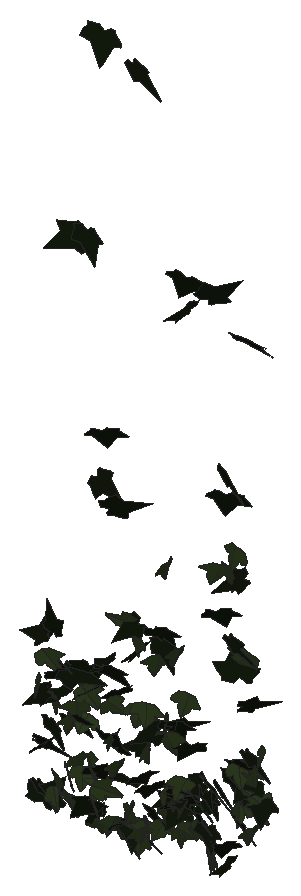
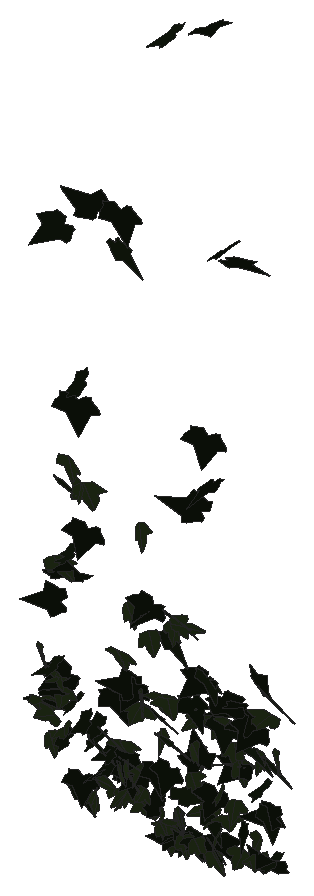
# SketchUp Ruby script. Lengths in inches.
U = 1.inch
M = Sketchup.active_model
def pt(a) = Geom::Point3d.new(a.map { |v| v * U })
def face(e, loops, mat)
  f = e.add_face(loops[0].map { |a| pt(a) })
  loops[1..].each { |l| e.add_face(l.map { |a| pt(a) }).erase! }
  f.material = f.back_material = mat if mat
  f
end
# faces: each face lists its corners as indices into pts; further lists are holes
def faces(e, pts, list, mat = nil) = list.each { |f| face(e, (f[0].is_a?(Array) ? f : [f]).map { |l| l.map { |i| pts[i] } }, mat) }
# xy, xz, yz: faces in a plane at the given z, y or x. An outline is a flat list of corners, or four numbers for a rectangle; further outlines are holes
def ring(l) = l.size == 4 ? [[l[0], l[1]], [l[2], l[1]], [l[2], l[3]], [l[0], l[3]]] : l.each_slice(2).to_a
def flat(e, list, mat, &to3) = list.each { |f| face(e, (f[0].is_a?(Array) ? f : [f]).map { |l| ring(l).map { |u, v| to3.(u, v) } }, mat) }
def xy(e, z, list, mat = nil) = flat(e, list, mat) { |x, y| [x, y, z] }
def xz(e, y, list, mat = nil) = flat(e, list, mat) { |x, z| [x, y, z] }
def yz(e, x, list, mat = nil) = flat(e, list, mat) { |y, z| [x, y, z] }
def lines(e, pts, list) = list.each { |a, b| e.add_line(pt(pts[a]), pt(pts[b])) }
# prism: a flat outline (further loops are holes) pulled along v
def prism(e, loops, v, mat = nil)
  f = face(e, loops, mat); d = Geom::Vector3d.new(v.map { |x| x * U })
  f.pushpull(f.normal.samedirection?(d) ? d.length : -d.length)
end
def box(e, o, s, mat = nil) = prism(e, [[o, [o[0] + s[0], o[1], o[2]], [o[0] + s[0], o[1] + s[1], o[2]], [o[0], o[1] + s[1], o[2]]]], [0, 0, s[2]], mat)
def at(x, y, z, deg = 0) = Geom::Transformation.translation(pt([x, y, z])) * Geom::Transformation.rotation(ORIGIN, Z_AXIS, deg.degrees)
def axes(o, x, y, z) = Geom::Transformation.new([*x, 0, *y, 0, *z, 0, *pt(o).to_a, 1])
def part(name) = M.definitions.add(name)
# library, detail: a bought-in or finely detailed component or shape, given as its bounding box
def library(name, o, s) = part(name).tap { |d| box(d.entities, o, s) }
def detail(e, o, s) = box(e.add_group.entities, o, s)
def put(e, d, t, mat = nil) = e.add_instance(d, t).tap { |i| i.material = mat if mat }
def group(e, t, mat = nil) = e.add_group.tap { |g| g.transformation = t; g.material = mat if mat }.entities
root = M.entities
M.materials.add("1026 AP 7946 SUNNY SIDE UP").color = [254, 231, 186]
M.materials.add("efeu1").color = [18, 25, 13]
M.materials.add("efeu2").color = [43, 57, 29]
c1 = part("ivyleaf_10")
p = [[0,0.5,-0.03],[-0.0625,2.02,-0.43],[-0.19,2.01,-0.46],[-0.54,1.05,-0.29],[-0.52,0.625,-0.18],[-0.83,0.76,-0.28],
  [-1.16,0.64,-0.33],[-1.15,0.33,-0.24],[-0.77,-0.39,0.02],[-0.3,-0.51,0.16],[0.04,-0.48,0.23],[-0.02,2.01,-0.4375],
  [-0.06,2.01,-0.43],[0.04,-0.49,0.23],[0.67,-0.49,0.14],[1.38,0.36,-0.2],[1.375,0.51,-0.24],[0.81,0.65,-0.19],
  [0.62,0.59,-0.15],[0.6,1.09,-0.28],[0.5,1.23,-0.31]]
faces(c1.entities,p,[[0,1,2,3,4,5,6,7,8,9,10],[11,12,0,13,14,15,16,17,18,19,20]],"efeu2")
c2 = part("ivyleaf_9")
p = [[1.54,2.16,1.25],[1.36,2.04,1.19],[-0.21,0.99,0.68],[-0.71,1.11,0.82],[-0.85,0.86,0.67],[-0.8,0.17,0.21],
  [-0.9,-0.01,0.1],[-0.67,-0.16,-0.02],[-0.08,-0.08,-0.05],[-0.03,-0.6,-0.4],[0.65,-0.88,-0.66],[0.83,-0.6,-0.49],
  [1.29,-0.42,-0.43],[1.8125,-0.07,-0.26],[1.21,0.44,0.15]]
faces(c2.entities,p,[[0,1,2,3,4,5,6,7,8,9,10,11,12,13,14]],"efeu1")
put(root,c1,axes([141.1,212.78,296.36],[0.23401,-0.33975,0.03293],[0.06355,-0.01919,-0.38104],[0.53311,0.15142,0.03097]),"1026 AP 7946 SUNNY SIDE UP")
put(root,c2,axes([141.62,212.62,298.74],[-0.37048,0.27885,0.16056],[-0.19198,0.09823,-0.37444],[-0.46286,-0.26394,0.02679]),"1026 AP 7946 SUNNY SIDE UP")
put(root,c2,axes([141.55,212.71,295.99],[-0.47568,0.21969,-0.05236],[0.04177,-0.05181,-0.38453],[-0.35255,-0.30256,0.02508]),"1026 AP 7946 SUNNY SIDE UP")
put(root,c2,axes([141.46,212.6,293.67],[0.03178,0.37624,0.06452],[0.00068,0.06056,-0.3878],[-0.5992,0.02002,0.00298]),"1026 AP 7946 SUNNY SIDE UP")
put(root,c2,axes([141.19,212.7,291.74],[0.30088,-0.30778,0.01172],[0.04466,0.00224,-0.37243],[0.48233,0.19179,0.02717]),"1026 AP 7946 SUNNY SIDE UP")
put(root,c2,axes([141.18,212.74,293.68],[0.47621,-0.09909,0.19336],[0.29609,-0.02755,-0.32718],[0.15567,0.35553,0.0308]),"1026 AP 7946 SUNNY SIDE UP")
put(root,c2,axes([141.6,212.5,291.24],[-0.39293,0.07877,0.33366],[0.51009,-0.03309,0.26632],[0.11741,0.40738,-0.04039]),"1026 AP 7946 SUNNY SIDE UP")
put(root,c2,axes([142.01,212.58,299.02],[0.20564,-0.05326,0.38485],[-0.16988,0.37384,0.09598],[-0.569,-0.13086,0.11043]),"1026 AP 7946 SUNNY SIDE UP")
put(root,c1,axes([141.87,212.67,296],[-0.425,0.25859,-0.01348],[-0.00975,-0.02749,-0.38471],[-0.40713,-0.26928,0.02329]),"1026 AP 7946 SUNNY SIDE UP")
put(root,c1,axes([141.62,212.59,297.79],[0.41531,0.16583,0.22308],[0.23144,0.16559,-0.31599],[-0.35966,0.29804,0.05426]),"1026 AP 7946 SUNNY SIDE UP")
put(root,c2,axes([142.32,212.61,296.15],[-0.1477,0.34832,0.13655],[-0.22561,0.09032,-0.35403],[-0.53965,-0.13309,0.11064]),"1026 AP 7946 SUNNY SIDE UP")
put(root,c2,axes([141.71,212.78,294.68],[0.21831,-0.33799,0.06151],[0.02425,-0.06027,-0.37668],[0.53968,0.13943,-0.00796]),"1026 AP 7946 SUNNY SIDE UP")
put(root,c1,axes([142.05,212.66,292.42],[-0.36108,0.27731,-0.08882],[0.05685,-0.08378,-0.37052],[-0.45383,-0.23113,0.02426]),"1026 AP 7946 SUNNY SIDE UP")
put(root,c1,axes([142.02,212.64,291.67],[0.21109,0.3459,-0.01846],[0.00948,-0.02366,-0.3821],[-0.54471,0.13363,-0.0138]),"1026 AP 7946 SUNNY SIDE UP")
put(root,c2,axes([142.16,212.63,297.15],[0.42578,0.2831,0.06142],[0.08605,0.02782,-0.40288],[-0.44617,0.27552,-0.0191]),"1026 AP 7946 SUNNY SIDE UP")
put(root,c2,axes([142.625,212.73,292.73],[0.27139,-0.07076,-0.33383],[-0.46411,0.13287,-0.19131],[0.23656,0.34187,0.00765]),"1026 AP 7946 SUNNY SIDE UP")
put(root,c2,axes([142.33,212.76,297.41],[0.50286,-0.18869,0.07094],[0.07479,-0.05672,-0.38205],[0.30745,0.32241,-0.0231]),"1026 AP 7946 SUNNY SIDE UP")
put(root,c2,axes([143.08,212.96,317.11],[-0.61078,-0.11039,0.17032],[-0.23093,-0.08724,-0.41443],[0.21188,-0.4133,0.03929]),"1026 AP 7946 SUNNY SIDE UP")
put(root,c1,axes([142.76,212.78,291.6],[-0.54065,0.12301,-0.06348],[0.078,-0.04587,-0.37551],[-0.2023,-0.34642,0.02486]),"1026 AP 7946 SUNNY SIDE UP")
put(root,c1,axes([142.87,212.7,295.28],[-0.16138,-0.3596,0.04032],[0.00395,-0.04351,-0.38523],[0.56912,-0.10166,0.01411]),"1026 AP 7946 SUNNY SIDE UP")
put(root,c1,axes([143.14,212.6875,295.99],[-0.37724,-0.29186,0.02678],[0.0498,-0.06133,-0.38408],[0.45827,-0.23359,0.06379]),"1026 AP 7946 SUNNY SIDE UP")
put(root,c1,axes([143.1,212.74,293.55],[-0.168,-0.32845,-0.12818],[0.09336,0.10932,-0.3545],[0.54327,-0.12036,0.02128]),"1026 AP 7946 SUNNY SIDE UP")
put(root,c2,axes([142.875,212.625,295.36],[0.58101,0.08974,-0.0109],[-0.00379,-0.03687,-0.39026],[-0.14213,0.36783,-0.03416]),"1026 AP 7946 SUNNY SIDE UP")
put(root,c2,axes([142.91,212.43,297.58],[0.21427,-0.06615,-0.38429],[0.18921,0.38309,-0.02248],[0.56424,-0.10334,0.15347]),"1026 AP 7946 SUNNY SIDE UP")
put(root,c2,axes([143.66,212.69,297.93],[0.04781,0.19675,-0.33736],[-0.2757,-0.2859,-0.19474],[-0.53539,0.16479,0.07016]),"1026 AP 7946 SUNNY SIDE UP")
put(root,c1,axes([143.36,213.01,295.32],[-0.54257,-0.07603,0.11791],[0.09183,-0.36135,-0.06778],[0.19621,-0.04114,0.35779]),"1026 AP 7946 SUNNY SIDE UP")
put(root,c1,axes([143.27,212.8125,292.99],[0.38602,0.26618,-0.03326],[-0.00107,-0.04518,-0.37202],[-0.4219,0.24366,-0.02948]),"1026 AP 7946 SUNNY SIDE UP")
put(root,c2,axes([143.67,212.64,296.78],[0.12735,0.38269,0.06794],[-0.00071,0.06524,-0.40235],[-0.61005,0.07981,0.01465]),"1026 AP 7946 SUNNY SIDE UP")
put(root,c2,axes([143.84,212.67,291.82],[0.1815,0.14723,-0.33719],[-0.28391,-0.27433,-0.19383],[-0.4891,0.21388,-0.01261]),"1026 AP 7946 SUNNY SIDE UP")
put(root,c2,axes([143.47,212.87,317.43],[0.03394,-0.43558,-0.00802],[-0.00435,0.00518,-0.44925],[0.68495,0.02161,-0.00246]),"1026 AP 7946 SUNNY SIDE UP")
put(root,c1,axes([144.15,212.75,291.03],[-0.32602,0.06883,0.2946],[-0.44153,0.05622,-0.22365],[-0.13566,-0.3484,0.01994]),"1026 AP 7946 SUNNY SIDE UP")
put(root,c1,axes([143.6,212.58,296.84],[0.33705,0.26963,0.20856],[0.15988,0.17513,-0.35286],[-0.50397,0.23588,0.02753]),"1026 AP 7946 SUNNY SIDE UP")
put(root,c2,axes([144.09,212.61,291.27],[0.00331,0.20768,0.31229],[-0.10085,0.29751,-0.2086],[-0.56736,-0.05167,0.0389]),"1026 AP 7946 SUNNY SIDE UP")
put(root,c1,axes([143.88,212.6,293.82],[-0.14166,0.37381,-0.04572],[0.00415,-0.04719,-0.3963],[-0.5923,-0.08973,0.00816]),"1026 AP 7946 SUNNY SIDE UP")
put(root,c1,axes([143.94,212.67,292.03],[-0.22459,0.3481,0.0411],[-0.03112,0.03286,-0.38739],[-0.54971,-0.14408,0.00514]),"1026 AP 7946 SUNNY SIDE UP")
put(root,c2,axes([144.35,212.65,292.57],[-0.13934,0.35776,0.01186],[-0.00059,0.00967,-0.37964],[-0.56275,-0.0886,-0.00254]),"1026 AP 7946 SUNNY SIDE UP")
put(root,c1,axes([144.07,212.91,292.52],[-0.35547,-0.112,0.26594],[0.18891,-0.33833,-0.0447],[0.40113,0.06008,0.25672]),"1026 AP 7946 SUNNY SIDE UP")
put(root,c2,axes([144.2,212.5,293.57],[0.33751,0.30228,0.00072],[0.02164,-0.01102,-0.38157],[-0.47482,0.21437,-0.01688]),"1026 AP 7946 SUNNY SIDE UP")
put(root,c2,axes([144.6,212.51,298.38],[-0.04896,0.34709,0.17645],[-0.12136,0.16084,-0.35336],[-0.59498,-0.06136,0.05756]),"1026 AP 7946 SUNNY SIDE UP")
put(root,c2,axes([144.29,212.89,326.76],[-0.21705,-0.4431,0.01108],[0.01233,-0.01633,-0.47804],[0.69694,-0.13771,0.01191]),"1026 AP 7946 SUNNY SIDE UP")
put(root,c2,axes([144.51,212.61,308.89],[0.40007,0.31603,-0.11319],[-0.08902,-0.09766,-0.4182],[-0.51946,0.26013,-0.01551]),"1026 AP 7946 SUNNY SIDE UP")
put(root,c2,axes([144.41,212.46,306.82],[0.2162,-0.22829,-0.35325],[-0.17454,0.32619,-0.26869],[0.62202,0.17088,0.04739]),"1026 AP 7946 SUNNY SIDE UP")
put(root,c1,axes([144.44,212.41,292.8],[0.14338,0.10974,0.36927],[0.28065,0.31096,-0.14328],[-0.51727,0.19913,0.02461]),"1026 AP 7946 SUNNY SIDE UP")
put(root,c1,axes([144.86,212.81,291.32],[-0.19254,-0.32295,0.09826],[0.00317,-0.10412,-0.35433],[0.5303,-0.11663,0.03779]),"1026 AP 7946 SUNNY SIDE UP")
put(root,c1,axes([145.02,212.7,295.29],[0.03373,-0.3882,0.0273],[-0.02043,-0.02944,-0.40043],[0.61174,0.02042,-0.01487]),"1026 AP 7946 SUNNY SIDE UP")
put(root,c2,axes([144.71,212.47,298.3],[0.58479,0.106,0.02136],[0.03494,-0.00452,-0.39828],[-0.16601,0.37243,-0.00856]),"1026 AP 7946 SUNNY SIDE UP")
put(root,c2,axes([144.7,212.8,294.81],[0.62008,-0.13382,-0.04098],[0.07829,0.02587,0.42715],[-0.20473,-0.39543,0.03923]),"1026 AP 7946 SUNNY SIDE UP")
put(root,c2,axes([145.17,212.72,297.31],[0.00488,0.35768,-0.13712],[-0.00408,-0.13511,-0.36928],[-0.6012,0.00382,0.00139]),"1026 AP 7946 SUNNY SIDE UP")
put(root,c1,axes([144.87,212.62,296.74],[-0.23401,-0.24633,-0.25598],[0.30626,0.1642,-0.28855],[0.45515,-0.23714,0.06255]),"1026 AP 7946 SUNNY SIDE UP")
put(root,c1,axes([145.17,212.6875,294.03],[-0.06862,-0.36447,0.0429],[0.00619,-0.04448,-0.3783],[0.57716,-0.04285,0.00916]),"1026 AP 7946 SUNNY SIDE UP")
put(root,c2,axes([145.53,212.62,291.48],[-0.05143,0.32818,-0.14031],[-0.13426,-0.14183,-0.3273],[-0.5435,0.00398,0.09413]),"1026 AP 7946 SUNNY SIDE UP")
put(root,c1,axes([145.73,212.86,300.47],[-0.02821,-0.0392,-0.39678],[-0.60516,0.04144,0.01437],[0.06258,0.38311,-0.03986]),"1026 AP 7946 SUNNY SIDE UP")
put(root,c2,axes([145.41,213.11,293.21],[-0.52004,-0.09222,0.12021],[0.09845,-0.34464,-0.09935],[0.21284,-0.0659,0.33967]),"1026 AP 7946 SUNNY SIDE UP")
put(root,c2,axes([144.91,212.625,305.54],[0.18396,0.00479,0.42982],[0.64521,0.0771,-0.11901],[-0.11874,0.42638,0.01926]),"1026 AP 7946 SUNNY SIDE UP")
put(root,c1,axes([145.45,212.86,291.32],[-0.17543,-0.33921,0.00432],[0.00595,-0.00769,-0.36786],[0.53343,-0.11147,0.00552]),"1026 AP 7946 SUNNY SIDE UP")
put(root,c1,axes([145.8,212.66,292.15],[-0.40458,0.23715,0.08461],[-0.2029,-0.02618,-0.34436],[-0.33767,-0.26841,0.10554]),"1026 AP 7946 SUNNY SIDE UP")
put(root,c2,axes([145.42,212.72,291.05],[0.33369,-0.28248,0.0278],[0.00101,-0.03521,-0.36357],[0.44644,0.21122,-0.01995]),"1026 AP 7946 SUNNY SIDE UP")
put(root,c1,axes([145.77,212.8,292.22],[0.16406,-0.34717,-0.00325],[0.00489,0.00217,-0.37342],[0.54587,0.10432,0.00432]),"1026 AP 7946 SUNNY SIDE UP")
put(root,c2,axes([146.07,212.78,300.65],[-0.59885,0.06002,-0.07322],[0.09826,-0.05872,-0.39451],[-0.1089,-0.38301,0.04666]),"1026 AP 7946 SUNNY SIDE UP")
put(root,c2,axes([145.76,212.9,291.32],[-0.13415,-0.34495,-0.00058],[0.0153,-0.00385,-0.36594],[0.54218,-0.08524,0.01018]),"1026 AP 7946 SUNNY SIDE UP")
put(root,c1,axes([146.08,212.71,300.07],[-0.4731,0.24291,0.01248],[-0.06813,-0.03676,-0.39442],[-0.37621,-0.29882,0.05574]),"1026 AP 7946 SUNNY SIDE UP")
put(root,c2,axes([146.38,212.61,299.62],[-0.2777,0.34324,-0.07027],[0.02868,-0.06946,-0.39776],[-0.55012,-0.17689,0.01474]),"1026 AP 7946 SUNNY SIDE UP")
put(root,c2,axes([146.51,212.81,295.32],[-0.44878,0.23479,0.0577],[-0.15145,-0.03339,-0.37047],[-0.3475,-0.28868,0.08695]),"1026 AP 7946 SUNNY SIDE UP")
put(root,c1,axes([146.2,212.92,291.6],[0.55211,0.03416,0.00959],[0.0191,-0.03116,-0.3621],[-0.0522,0.34986,-0.03111]),"1026 AP 7946 SUNNY SIDE UP")
put(root,c1,axes([146.27,212.71,296.87],[0.52607,0.16942,-0.0425],[-0.08687,0.01615,-0.38414],[-0.26044,0.33683,0.04227]),"1026 AP 7946 SUNNY SIDE UP")
put(root,c2,axes([146.34,212.59,293.89],[0.20092,0.34654,0.06261],[0.05113,0.05065,-0.37998],[-0.55032,0.13123,-0.01244]),"1026 AP 7946 SUNNY SIDE UP")
put(root,c2,axes([145.96,212.82,325.83],[0.39448,-0.38327,-0.07328],[0.0021,0.08288,-0.46904],[0.61233,0.24663,0.04882]),"1026 AP 7946 SUNNY SIDE UP")
put(root,c1,axes([146.27,212.76,291.02],[0.52057,-0.1196,0.00923],[0.03122,0.02671,-0.36099],[0.18606,0.33013,0.03475]),"1026 AP 7946 SUNNY SIDE UP")
put(root,c2,axes([145.97,212.93,291.24],[0.38619,-0.20963,0.14912],[0.16795,-0.09962,-0.33318],[0.36484,0.26776,-0.00447]),"1026 AP 7946 SUNNY SIDE UP")
put(root,c1,axes([146.4,212.91,291.6],[-0.20847,-0.28724,0.16596],[0.05425,-0.18645,-0.31119],[0.51625,-0.0964,0.09972]),"1026 AP 7946 SUNNY SIDE UP")
put(root,c1,axes([146.43,212.63,291.48],[-0.18664,-0.33884,-0.08269],[0.06671,0.06806,-0.36905],[0.54276,-0.12488,0.01692]),"1026 AP 7946 SUNNY SIDE UP")
put(root,c1,axes([146.53,212.81,291.88],[-0.14403,0.26578,-0.22107],[0.09572,-0.2075,-0.29071],[-0.53004,-0.1097,0.00757]),"1026 AP 7946 SUNNY SIDE UP")
put(root,c1,axes([146.53,212.76,297.02],[0.53887,0.15858,0.01228],[0.04061,-0.0297,-0.38724],[-0.24663,0.34159,-0.03692]),"1026 AP 7946 SUNNY SIDE UP")
put(root,c1,axes([146.7,212.6,295.27],[0.08349,-0.36142,-0.10225],[0.10702,0.10586,-0.36658],[0.57867,0.03257,0.08255]),"1026 AP 7946 SUNNY SIDE UP")
put(root,c2,axes([146.95,212.57,293.7],[0.09888,0.35874,-0.09157],[-0.02245,-0.08981,-0.37573],[-0.58149,0.06447,-0.00107]),"1026 AP 7946 SUNNY SIDE UP")
put(root,c2,axes([147.22,212.68,296.23],[-0.55489,0.1257,-0.00833],[-0.00379,-0.03289,-0.38472],[-0.1981,-0.35147,0.03068]),"1026 AP 7946 SUNNY SIDE UP")
put(root,c1,axes([147.16,212.76,299.43],[-0.29926,-0.33535,0.04431],[0.00555,-0.05349,-0.3964],[0.53198,-0.18809,0.02906]),"1026 AP 7946 SUNNY SIDE UP")
put(root,c2,axes([146.73,212.85,292.25],[0.30208,-0.17398,0.25785],[0.25597,-0.19295,-0.26697],[0.40674,0.25064,-0.0235]),"1026 AP 7946 SUNNY SIDE UP")
put(root,c2,axes([147.14,212.67,300.77],[0.55033,0.17405,-0.01399],[0.00254,-0.03585,-0.40147],[-0.27461,0.34846,-0.03175]),"1026 AP 7946 SUNNY SIDE UP")
put(root,c1,axes([147.46,212.7,292.05],[0.36612,0.22246,-0.15451],[-0.21374,-0.07531,-0.33015],[-0.36499,0.26724,0.03835]),"1026 AP 7946 SUNNY SIDE UP")
put(root,c1,axes([147.53,212.82,296.74],[0.21494,-0.34187,-0.08438],[0.03784,0.09473,-0.3743],[0.55077,0.12691,0.05864]),"1026 AP 7946 SUNNY SIDE UP")
put(root,c1,axes([147.59,212.77,303.89],[-0.00162,-0.39303,-0.08643],[0.02642,0.08156,-0.40407],[0.63065,-0.00442,0.01671]),"1026 AP 7946 SUNNY SIDE UP")
put(root,c1,axes([147.49,212.81,292.7],[-0.47499,0.14365,-0.13126],[0.12007,-0.12964,-0.33568],[-0.27795,-0.30148,0.07931]),"1026 AP 7946 SUNNY SIDE UP")
put(root,c2,axes([147.39,212.72,300.28],[0.11439,-0.37784,-0.08436],[-0.03287,0.07717,-0.3959],[0.60632,0.07547,-0.00555]),"1026 AP 7946 SUNNY SIDE UP")
put(root,c1,axes([147.62,212.67,293.5],[0.01662,0.32108,0.18296],[-0.04912,0.17599,-0.32823],[-0.57347,-0.00577,0.03341]),"1026 AP 7946 SUNNY SIDE UP")
put(root,c1,axes([147.71,212.73,296.14],[-0.52798,-0.14396,-0.1082],[0.18419,-0.01175,-0.37218],[0.21015,-0.35138,0.05437]),"1026 AP 7946 SUNNY SIDE UP")
put(root,c2,axes([147.6,212.77,293.39],[0.56634,-0.01902,-0.05095],[-0.07883,-0.01454,-0.37124],[0.0265,0.36325,-0.0154]),"1026 AP 7946 SUNNY SIDE UP")
put(root,c2,axes([148.23,212.79,293.62],[-0.55372,0.07287,-0.00449],[-0.01887,-0.08092,-0.36126],[-0.11326,-0.34276,0.08212]),"1026 AP 7946 SUNNY SIDE UP")
put(root,c1,axes([147.73,212.92,292.76],[0.23634,-0.20809,-0.26063],[0.27422,-0.18326,0.26218],[-0.43432,-0.22894,0.02371]),"1026 AP 7946 SUNNY SIDE UP")
put(root,c2,axes([148.16,212.62,293.27],[0.19957,0.32556,-0.08514],[-0.04997,-0.07829,-0.36043],[-0.5265,0.13083,0.00194]),"1026 AP 7946 SUNNY SIDE UP")
put(root,c1,axes([148.14,212.82,293.49],[0.02818,-0.36452,0.02831],[-0.00707,-0.02981,-0.3761],[0.575,0.0175,-0.00601]),"1026 AP 7946 SUNNY SIDE UP")
put(root,c2,axes([148.03,212.54,296.9],[0.48192,0.21837,-0.05451],[-0.05176,-0.047,-0.38747],[-0.34996,0.30766,-0.01775]),"1026 AP 7946 SUNNY SIDE UP")
put(root,c1,axes([148.23,212.6875,300.22],[-0.03132,-0.38972,0.04383],[-0.00071,-0.0448,-0.40227],[0.61682,-0.01984,0.00176]),"1026 AP 7946 SUNNY SIDE UP")
put(root,c2,axes([148.26,212.85,293.05],[-0.41502,-0.24429,0.0288],[-0.00743,-0.03799,-0.36986],[0.38681,-0.26284,0.02379]),"1026 AP 7946 SUNNY SIDE UP")
put(root,c2,axes([148.68,212.8,315.76],[-0.36029,0.3663,-0.06952],[-0.01338,-0.08677,-0.44231],[-0.58611,-0.22319,0.05283]),"1026 AP 7946 SUNNY SIDE UP")
put(root,c1,axes([148.4,212.93,293.27],[0.16405,-0.33587,0.08391],[0.01717,-0.08383,-0.36252],[0.54388,0.10395,-0.01387]),"1026 AP 7946 SUNNY SIDE UP")
put(root,c2,axes([148.35,212.625,293.83],[0.50851,0.12069,-0.14982],[-0.20235,-0.07229,-0.35538],[-0.21875,0.34743,-0.01953]),"1026 AP 7946 SUNNY SIDE UP")
put(root,c2,axes([148.1,212.59,296.81],[0.28654,0.02095,0.34627],[0.46586,0.17146,-0.17555],[-0.25138,0.34162,0.06938]),"1026 AP 7946 SUNNY SIDE UP")
put(root,c2,axes([148.61,212.7,317.23],[0.45722,0.13536,-0.31566],[-0.40702,-0.16832,-0.32983],[-0.33605,0.38804,-0.02999]),"1026 AP 7946 SUNNY SIDE UP")
put(root,c1,axes([148.43,212.61,292.03],[0.11403,-0.16502,-0.3243],[0.11549,0.3204,-0.15419],[0.54548,-0.03334,0.10043]),"1026 AP 7946 SUNNY SIDE UP")
put(root,c1,axes([148.37,212.65,292.21],[-0.19902,-0.22848,-0.25888],[0.25901,0.19166,-0.26525],[0.46531,-0.20441,0.03692]),"1026 AP 7946 SUNNY SIDE UP")
put(root,c1,axes([148.5,212.72,294.32],[0.56444,0.066,-0.07777],[-0.10302,-0.05982,-0.37336],[-0.11994,0.36199,-0.04527]),"1026 AP 7946 SUNNY SIDE UP")
put(root,c1,axes([148.59,212.78,298.18],[0.59659,-0.05307,0.00325],[-0.00336,-0.04008,-0.39275],[0.08356,0.37731,-0.03899]),"1026 AP 7946 SUNNY SIDE UP")
put(root,c2,axes([148.96,212.58,296.23],[0.09605,0.31868,-0.20662],[-0.09803,-0.19367,-0.33471],[-0.58545,0.08471,0.02215]),"1026 AP 7946 SUNNY SIDE UP")
put(root,c2,axes([149.28,212.83,294.52],[-0.53288,0.13821,-0.04917],[0.05731,-0.03888,-0.37659],[-0.22308,-0.34014,0.02072]),"1026 AP 7946 SUNNY SIDE UP")
put(root,c2,axes([148.9,212.81,293.87],[0.40364,-0.25376,0.01928],[0.00062,-0.02822,-0.37146],[0.40027,0.25594,-0.01886]),"1026 AP 7946 SUNNY SIDE UP")
put(root,c2,axes([149,212.74,293.27],[0.41632,-0.23361,-0.07923],[-0.10205,0.04062,-0.3633],[0.37234,0.27233,-0.01098]),"1026 AP 7946 SUNNY SIDE UP")
put(root,c1,axes([148.96,212.89,292.38],[-0.13846,-0.00201,-0.35908],[0.41663,-0.23395,-0.06894],[-0.35608,-0.27295,0.05896]),"1026 AP 7946 SUNNY SIDE UP")
put(root,c2,axes([149.91,212.75,293.95],[-0.47854,0.19099,-0.05006],[0.04677,-0.04588,-0.36967],[-0.30676,-0.30493,0.02174]),"1026 AP 7946 SUNNY SIDE UP")
put(root,c1,axes([149.8,212.78,291.5],[-0.39281,0.26094,0.01172],[-0.09823,-0.04643,-0.36382],[-0.39867,-0.24566,0.0781]),"1026 AP 7946 SUNNY SIDE UP")
put(root,c2,axes([149.64,212.82,292.64],[-0.01987,-0.36159,0.02921],[0.00033,-0.03044,-0.37291],[0.57056,-0.01258,0.00123]),"1026 AP 7946 SUNNY SIDE UP")
put(root,c2,axes([149.56,212.93,294.13],[0.12362,-0.33763,0.1045],[0.05084,-0.09856,-0.35759],[0.55288,0.08455,0.00952]),"1026 AP 7946 SUNNY SIDE UP")
put(root,c1,axes([149.86,212.73,291.75],[-0.10308,0.34779,-0.08273],[0.00855,-0.08267,-0.36495],[-0.5619,-0.06506,0.00962]),"1026 AP 7946 SUNNY SIDE UP")
put(root,c2,axes([149.58,212.82,294.68],[0.36161,-0.27054,0.10729],[0.10618,-0.0813,-0.36627],[0.44419,0.23968,0.00022]),"1026 AP 7946 SUNNY SIDE UP")
put(root,c1,axes([150.29,212.73,304.68],[-0.43309,-0.2668,0.12388],[-0.11345,-0.10027,-0.39505],[0.44697,-0.28397,0.01977]),"1026 AP 7946 SUNNY SIDE UP")
put(root,c2,axes([149.87,212.66,316.81],[-0.03207,-0.09234,0.4444],[0.66978,0.11013,0.04562],[-0.1835,0.41812,0.08886]),"1026 AP 7946 SUNNY SIDE UP")
put(root,c2,axes([150.43,212.73,292.18],[0.21496,0.32903,-0.08011],[-0.03371,-0.07729,-0.36737],[-0.53123,0.13804,-0.0091]),"1026 AP 7946 SUNNY SIDE UP")
put(root,c2,axes([150.36,212.53,302.8],[0.39903,0.30264,-0.05985],[-0.03845,-0.05747,-0.40679],[-0.48355,0.25431,-0.01704]),"1026 AP 7946 SUNNY SIDE UP")
put(root,c2,axes([150.14,212.78,294.74],[0.42314,-0.24297,-0.04737],[-0.08845,0.00395,-0.37179],[0.37822,0.27275,-0.03395]),"1026 AP 7946 SUNNY SIDE UP")
put(root,c2,axes([150.92,212.58,291.52],[-0.33097,0.29206,-0.05157],[0.01986,-0.05453,-0.37054],[-0.46596,-0.20977,0.02084]),"1026 AP 7946 SUNNY SIDE UP")
put(root,c1,axes([150.55,212.82,304.7],[-0.36988,0.27584,-0.17605],[0.1259,-0.15718,-0.37243],[-0.49579,-0.24571,0.03677]),"1026 AP 7946 SUNNY SIDE UP")
put(root,c2,axes([150.77,212.58,308.21],[0.43752,0.26393,-0.21882],[-0.20873,-0.17004,-0.39504],[-0.49172,0.30703,-0.02701]),"1026 AP 7946 SUNNY SIDE UP")
put(root,c2,axes([150.51,212.625,309.17],[0.48936,-0.29724,-0.09537],[-0.13586,0.04082,-0.44207],[0.46948,0.32164,-0.02852]),"1026 AP 7946 SUNNY SIDE UP")
put(root,c1,axes([151.05,212.85,305.64],[-0.56838,0.17611,0.04426],[-0.16414,-0.12618,-0.38152],[-0.23259,-0.34133,0.16108]),"1026 AP 7946 SUNNY SIDE UP")
put(root,c2,axes([150.67,212.9,295.36],[0.20485,-0.34213,0.05071],[0.00612,-0.05322,-0.37714],[0.54392,0.12945,-0.01485]),"1026 AP 7946 SUNNY SIDE UP")
put(root,c2,axes([151.44,212.75,304.57],[-0.58328,0.14727,-0.05388],[0.01983,-0.10811,-0.39998],[-0.24539,-0.3588,0.09576]),"1026 AP 7946 SUNNY SIDE UP")
put(root,c1,axes([151.21,212.875,294.09],[0.09079,0.33084,-0.1475],[-0.03978,-0.14284,-0.34681],[-0.56662,0.06304,0.00071]),"1026 AP 7946 SUNNY SIDE UP")
put(root,c2,axes([150.95,212.7,301.65],[0.38042,-0.31282,-0.04464],[0.04374,0.0733,-0.40117],[0.49427,0.23428,0.06986]),"1026 AP 7946 SUNNY SIDE UP")
put(root,c1,axes([151.63,212.79,301.1],[-0.47113,-0.09292,0.2434],[-0.3038,-0.15484,-0.31537],[0.26016,-0.3491,0.07251]),"1026 AP 7946 SUNNY SIDE UP")
put(root,c2,axes([151.49,212.48,300.35],[-0.63911,-0.07398,0.18856],[0.26967,0.07711,0.42393],[-0.155,0.43922,-0.03995]),"1026 AP 7946 SUNNY SIDE UP")
put(root,c1,axes([151.4,212.74,295.66],[-0.5892,0.02554,0.00496],[-0.01116,-0.03576,-0.38534],[-0.03927,-0.37303,0.03506]),"1026 AP 7946 SUNNY SIDE UP")
put(root,c2,axes([151.12,212.79,293.61],[0.32545,-0.29034,0.0914],[0.06493,-0.08147,-0.36755],[0.4737,0.21064,-0.01242]),"1026 AP 7946 SUNNY SIDE UP")
put(root,c1,axes([151.33,212.66,296],[0.40404,0.26445,0.00836],[0.04558,-0.01898,-0.37835],[-0.41345,0.25634,-0.03354]),"1026 AP 7946 SUNNY SIDE UP")
put(root,c2,axes([151.25,212.5625,296.28],[0.58111,0.05731,0.04591],[0.06402,0.02576,-0.38462],[-0.09412,0.37131,0.02183]),"1026 AP 7946 SUNNY SIDE UP")
put(root,c2,axes([151.83,212.89,295.45],[-0.49344,-0.19207,0.00204],[0.01873,-0.02533,-0.3781],[0.30148,-0.3128,0.02683]),"1026 AP 7946 SUNNY SIDE UP")
put(root,c1,axes([151.73,212.8,296.14],[-0.5092,0.15429,-0.0855],[0.08377,-0.08133,-0.36653],[-0.26312,-0.32448,0.04877]),"1026 AP 7946 SUNNY SIDE UP")
put(root,c2,axes([151.52,212.59,315.57],[0.69299,0.03089,-0.00815],[-0.02167,0.08299,-0.44641],[-0.0453,0.43291,0.0888]),"1026 AP 7946 SUNNY SIDE UP")
put(root,c1,axes([151.94,212.71,293.39],[-0.08642,-0.36551,-0.00067],[0.00217,-0.00165,-0.38078],[0.57473,-0.05495,0.00134]),"1026 AP 7946 SUNNY SIDE UP")
put(root,c2,axes([151.64,212.83,296.64],[0.35333,-0.29881,-0.04844],[0.01304,0.06255,-0.38213],[0.47504,0.22053,0.04652]),"1026 AP 7946 SUNNY SIDE UP")
put(root,c2,axes([151.85,212.38,299.11],[0.32151,0.05873,0.3604],[0.45766,0.20238,-0.20928],[-0.31794,0.35071,0.06321]),"1026 AP 7946 SUNNY SIDE UP")
put(root,c1,axes([152.43,212.78,294.67],[0.25484,0.22449,0.25642],[-0.26608,-0.18222,0.28321],[0.45323,-0.2332,0.02209]),"1026 AP 7946 SUNNY SIDE UP")
put(root,c1,axes([151.84,212.82,294.42],[0.33606,0.0049,0.31034],[0.47258,0.02197,-0.21992],[-0.03263,0.36868,0.01115]),"1026 AP 7946 SUNNY SIDE UP")
put(root,c1,axes([152.4,212.8,297.01],[0.29548,-0.32845,0.01533],[0.02347,-0.01075,-0.38982],[0.51659,0.18836,0.00894]),"1026 AP 7946 SUNNY SIDE UP")
put(root,c2,axes([152.39,212.77,294.85],[-0.38262,-0.22605,-0.16776],[0.22469,0.08236,-0.33996],[0.37468,-0.28023,0.03255]),"1026 AP 7946 SUNNY SIDE UP")
